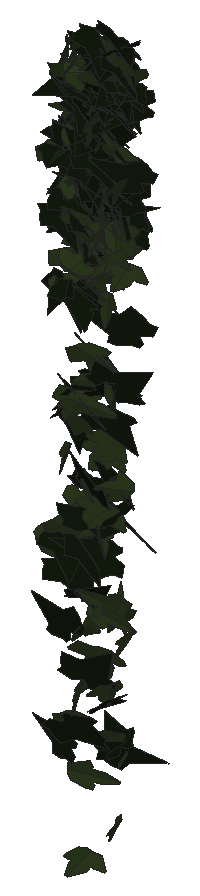
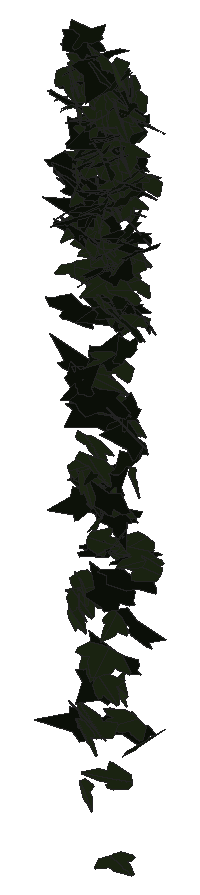
# SketchUp Ruby script. Lengths in millimetres.
U = 1.mm
M = Sketchup.active_model
def pt(a) = Geom::Point3d.new(a.map { |v| v * U })
def face(e, loops, mat)
  f = e.add_face(loops[0].map { |a| pt(a) })
  loops[1..].each { |l| e.add_face(l.map { |a| pt(a) }).erase! }
  f.material = f.back_material = mat if mat
  f
end
# faces: each face lists its corners as indices into pts; further lists are holes
def faces(e, pts, list, mat = nil) = list.each { |f| face(e, (f[0].is_a?(Array) ? f : [f]).map { |l| l.map { |i| pts[i] } }, mat) }
# xy, xz, yz: faces in a plane at the given z, y or x. An outline is a flat list of corners, or four numbers for a rectangle; further outlines are holes
def ring(l) = l.size == 4 ? [[l[0], l[1]], [l[2], l[1]], [l[2], l[3]], [l[0], l[3]]] : l.each_slice(2).to_a
def flat(e, list, mat, &to3) = list.each { |f| face(e, (f[0].is_a?(Array) ? f : [f]).map { |l| ring(l).map { |u, v| to3.(u, v) } }, mat) }
def xy(e, z, list, mat = nil) = flat(e, list, mat) { |x, y| [x, y, z] }
def xz(e, y, list, mat = nil) = flat(e, list, mat) { |x, z| [x, y, z] }
def yz(e, x, list, mat = nil) = flat(e, list, mat) { |y, z| [x, y, z] }
def lines(e, pts, list) = list.each { |a, b| e.add_line(pt(pts[a]), pt(pts[b])) }
# prism: a flat outline (further loops are holes) pulled along v
def prism(e, loops, v, mat = nil)
  f = face(e, loops, mat); d = Geom::Vector3d.new(v.map { |x| x * U })
  f.pushpull(f.normal.samedirection?(d) ? d.length : -d.length)
end
def box(e, o, s, mat = nil) = prism(e, [[o, [o[0] + s[0], o[1], o[2]], [o[0] + s[0], o[1] + s[1], o[2]], [o[0], o[1] + s[1], o[2]]]], [0, 0, s[2]], mat)
def at(x, y, z, deg = 0) = Geom::Transformation.translation(pt([x, y, z])) * Geom::Transformation.rotation(ORIGIN, Z_AXIS, deg.degrees)
def axes(o, x, y, z) = Geom::Transformation.new([*x, 0, *y, 0, *z, 0, *pt(o).to_a, 1])
def part(name) = M.definitions.add(name)
# library, detail: a bought-in or finely detailed component or shape, given as its bounding box
def library(name, o, s) = part(name).tap { |d| box(d.entities, o, s) }
def detail(e, o, s) = box(e.add_group.entities, o, s)
def put(e, d, t, mat = nil) = e.add_instance(d, t).tap { |i| i.material = mat if mat }
def group(e, t, mat = nil) = e.add_group.tap { |g| g.transformation = t; g.material = mat if mat }.entities
root = M.entities
M.materials.add("efeu1").color = [18, 25, 13]
M.materials.add("efeu2").color = [43, 57, 29]
c1 = part("ivyleaf_10")
p = [[0,12.8,-0.8],[-1.5,51.3,-10.9],[-4.9,51,-11.6],[-13.6,26.5,-7.3],[-13.2,15.9,-4.6],[-21.1,19.3,-7.2],
  [-29.5,16.3,-8.3],[-29.2,8.3,-6.2],[-19.7,-9.8,0.5],[-7.6,-13,4],[1,-12.2,5.8],[-0.4,51.1,-11.1],
  [-1.5,51.1,-10.9],[1,-12.4,5.9],[16.9,-12.4,3.5],[35.1,9.1,-5.1],[35,12.9,-6.1],[20.5,16.4,-4.9],
  [15.8,15,-3.8],[15.3,27.6,-7.1],[12.8,31.3,-7.8]]
faces(c1.entities,p,[[0,1,2,3,4,5,6,7,8,9,10],[11,12,0,13,14,15,16,17,18,19,20]],"efeu2")
c2 = part("ivyleaf_9")
p = [[39.1,54.8,31.7],[34.5,51.8,30.2],[-5.3,25.2,17.3],[-17.9,28.3,20.9],[-21.6,21.7,17],[-20.2,4.3,5.3],
  [-22.9,-0.3,2.5],[-17.1,-4,-0.6],[-2,-2.1,-1.2],[-0.7,-15.4,-10.1],[16.6,-22.3,-16.7],[21.1,-15.1,-12.5],
  [32.7,-10.7,-11],[46.1,-1.8,-6.6],[30.8,11.2,3.8]]
faces(c2.entities,p,[[0,1,2,3,4,5,6,7,8,9,10,11,12,13,14]],"efeu1")
put(root,c1,axes([2423.7,959.7,428.7],[0.42918,-0.51053,0.64216],[0.55619,-0.57229,-0.55762],[1.4589,0.36837,0.02368]))
put(root,c1,axes([2519.9,950.3,1384],[0.10116,-0.81817,0.0626],[-0.0042,-0.06288,-0.81987],[1.56168,0.05283,-0.00626]))
put(root,c1,axes([2466.4,955.7,1470.6],[0.11764,-0.75177,0.34655],[0.10851,-0.34282,-0.75385],[1.57173,0.07993,0.02611]))
put(root,c1,axes([2417.6,948.7,1568.5],[0.34944,-0.81684,-0.06645],[-0.02225,0.06548,-0.83722],[1.55959,0.18395,0.00295]))
put(root,c1,axes([2484,949.2,779.4],[1.57579,-0.10908,-0.34609],[-0.65321,0.04451,-0.83512],[0.22422,0.89629,-0.00065]))
put(root,c2,axes([2498.1,963.2,1633.7],[-0.17423,-0.67542,0.52153],[0.47468,-0.5228,-0.63328],[1.55316,0.08401,0.25205]))
put(root,c2,axes([2432.3,955.2,696.6],[0.16667,-0.81995,-0.11019],[-0.02639,0.10933,-0.82461],[1.57434,0.08864,-0.00216]))
put(root,c2,axes([2431,945.6,1418.8],[-0.93455,0.09387,0.70212],[1.23515,-0.28279,0.49169],[0.54033,0.80878,0.09043]))
put(root,c2,axes([2453.5,951.6,1417.3],[0.09734,-0.79256,-0.34222],[0.10732,0.34515,-0.79093],[1.63949,0.02446,0.07209]))
put(root,c2,axes([2457.5,943.1,740.9],[-1.30236,0.01154,0.54128],[1.03011,-0.00582,0.68439],[0.0241,0.87248,-0.00259]))
put(root,c1,axes([2378.7,944.8,1402.3],[-0.69228,-0.44049,-0.55113],[1.01872,0.23167,-0.53843],[0.87478,-0.61838,0.19087]))
put(root,c2,axes([2395.2,960.7,689.2],[-0.40626,-0.83532,-0.06765],[0.01712,0.06753,-0.86213],[1.5949,-0.2135,-0.00798]))
put(root,c2,axes([2391.9,946,1405.4],[0.10948,-0.47721,-0.63361],[0.10888,0.63611,-0.4739],[1.50571,-0.0113,0.08034]))
put(root,c2,axes([2463,949.2,798.5],[0.52534,-0.53448,0.66931],[-0.43549,0.63163,0.59876],[-1.5709,-0.35384,0.05784]))
put(root,c2,axes([2443.5,948.4,460.5],[-0.91593,0.14357,0.66024],[1.12315,-0.30542,0.49658],[0.62621,0.75779,0.07505]))
put(root,c1,axes([2472.4,954.6,734.5],[-0.10834,0.7349,-0.30371],[0.05244,-0.30248,-0.73709],[-1.51248,-0.06313,-0.0038]))
put(root,c2,axes([2391.5,957.8,1156.9],[-1.14108,0.14142,-0.49329],[0.89744,-0.14744,-0.6154],[-0.38528,-0.76228,0.02751]))
put(root,c1,axes([2404.9,961.3,1356.8],[0.27602,-0.50452,0.59318],[1.0173,-0.37428,-0.44903],[1.07776,0.4825,0.27193]))
put(root,c2,axes([2425.7,958.2,1153],[-0.68074,-0.70087,-0.2783],[0.22525,0.25203,-0.78682],[1.41742,-0.37666,-0.00862]))
put(root,c1,axes([2425.3,947,927.3],[-1.31838,0.29849,0.21379],[-0.37768,0.07971,-0.75428],[-0.58792,-0.72056,0.00512]))
put(root,c2,axes([2463,963.2,1620.2],[-0.43825,-0.82502,0.03105],[-0.0162,-0.02986,-0.85655],[1.5712,-0.23043,-0.00017]))
put(root,c1,axes([2477.4,960,1153.1],[1.04945,-0.44206,0.40539],[0.56454,-0.27763,-0.70622],[0.99216,0.62555,-0.02696]))
put(root,c2,axes([2403.1,957.8,317.2],[-0.23314,-0.79978,0.1421],[0.04083,0.14047,0.80911],[-1.54544,0.12436,-0.00006]))
put(root,c2,axes([2415.9,942.2,540.3],[-0.18859,0.13593,0.84531],[-0.87282,0.71015,-0.16795],[-1.37598,-0.4691,-0.00932]))
put(root,c1,axes([2520.4,950.6,1287.2],[1.16434,-0.44278,-0.34263],[-0.48377,0.23253,-0.75435],[0.94939,0.66152,0.03583]))
put(root,c1,axes([2509.7,965.4,816.4],[0.0865,0.23688,0.7628],[-0.26221,-0.75026,0.24119],[1.49736,-0.14506,-0.00183]))
put(root,c1,axes([2465,960.9,1303.9],[-0.40203,0.57267,-0.58428],[0.24087,-0.57331,-0.60767],[-1.53832,-0.23943,0.05755]))
put(root,c1,axes([2489.5,951,457.1],[-0.56264,-0.72009,-0.13796],[0.1065,0.12615,-0.7784],[1.39133,-0.30085,0.00379]))
put(root,c1,axes([2461.3,952,1485.8],[0.26626,-0.80695,-0.17252],[-0.0737,0.16837,-0.81893],[1.56876,0.14487,-0.00919]))
put(root,c1,axes([2445.5,960.7,1392.9],[0.75294,-0.71526,0.2599],[0.22999,-0.23016,-0.81736],[1.42998,0.41363,-0.00538]))
put(root,c1,axes([2399,955.6,1208.1],[-1.06414,-0.23857,-0.44204],[0.94713,-0.17329,-0.53596],[0.1298,-0.69137,0.28686]))
put(root,c2,axes([2517,941.3,782.8],[-0.34441,0.76154,0.32734],[-0.15165,0.31752,-0.78274],[-1.57028,-0.19769,0.0038]))
put(root,c1,axes([2457.3,961.4,1269.3],[0.82671,-0.61985,0.27564],[0.28301,-0.23234,-0.75682],[1.25968,0.459,-0.01087]))
put(root,c1,axes([2438.7,958.6,1473.2],[0.78386,-0.70817,0.08456],[0.0753,-0.07481,-0.81922],[1.35528,0.41374,-0.00339]))
put(root,c1,axes([2399.7,946,1405.5],[-0.13178,-0.61189,-0.50447],[0.12519,0.50021,-0.61575],[1.50409,-0.09524,0.00705]))
put(root,c1,axes([2485.9,958,1248.8],[0.84377,-0.22823,-0.69233],[1.21346,-0.27142,0.49776],[-0.67257,-0.77602,0.02952]))
put(root,c2,axes([2495.2,953,1000.4],[-0.60385,0.19408,0.80129],[1.31944,-0.40187,0.37185],[0.84922,0.76239,-0.00797]))
put(root,c2,axes([2500.2,966.4,1390.4],[-0.66734,0.06385,0.72928],[-1.15355,-0.47881,-0.2495],[0.78138,-0.65234,0.25451]))
put(root,c1,axes([2429,947.1,958.8],[-0.67269,-0.24827,-0.7794],[1.36217,0.3172,-0.42562],[0.75372,-0.79484,0.0736]))
put(root,c2,axes([2406.8,955.6,646.1],[-0.62425,-0.47585,-0.61472],[0.64503,0.51292,-0.57789],[1.3315,-0.47157,-0.00825]))
put(root,c1,axes([2419.8,963.3,1354.4],[0.11933,-0.74217,0.31287],[0.00074,-0.31379,-0.74442],[1.53287,0.05793,-0.024]))
put(root,c1,axes([2424.6,946.8,1202.8],[0.99733,0.27008,-0.47127],[0.68938,0.31422,0.58285],[0.77036,-0.63085,0.08854]))
put(root,c2,axes([2514.5,949,1626.2],[-0.04872,0.82399,-0.17062],[-0.02885,-0.17112,-0.82414],[-1.60122,-0.02199,0.02004]))
put(root,c2,axes([2403.7,969.9,952.3],[0.53392,-0.58906,0.69287],[0.5142,-0.63837,-0.65211],[1.65268,0.38892,-0.02095]))
put(root,c1,axes([2474.2,957.7,1611.6],[1.37264,-0.45576,-0.02408],[0.03134,0.07099,-0.85039],[0.86805,0.71813,0.06878]))
put(root,c1,axes([2501.8,958.1,212.5],[0.25989,-0.72766,-0.02306],[-0.00904,0.02257,-0.74036],[1.38554,0.13664,-0.0005]))
put(root,c2,axes([2452.4,966.5,1040.7],[0.95655,-0.66038,0.08772],[-0.09983,0.07031,0.82988],[-1.26393,-0.50533,0.00084]))
put(root,c2,axes([2405.7,948.5,365.1],[0.03186,-0.05946,-0.84196],[0.79779,0.73152,-0.04333],[1.39431,-0.4172,0.04403]))
put(root,c2,axes([2440.7,965.6,1376.1],[-0.18211,-0.80257,-0.06848],[0.01284,0.06816,-0.80825],[1.53294,-0.09592,-0.00137]))
put(root,c1,axes([2495.1,964.7,598.8],[-0.66578,-0.1313,-0.77141],[-1.36751,-0.28073,0.37362],[-0.58978,0.79915,0.00451]))
put(root,c2,axes([2376.4,961.5,1277.4],[0.16897,-0.78102,-0.2264],[0.00336,0.22793,-0.7856],[1.54762,0.08478,0.02643]))
put(root,c1,axes([2412.3,949.7,1559.7],[-1.04274,-0.30516,-0.59299],[0.94873,0.32242,-0.6265],[0.84315,-0.74018,-0.02842]))
put(root,c1,axes([2465.8,955.9,586],[0.43635,0.05961,0.75663],[1.39767,0.18218,-0.23688],[-0.36478,0.76933,-0.00253]))
put(root,c1,axes([2396.9,963.7,952.3],[1.11663,-0.49198,0.27184],[0.4082,-0.16726,-0.76563],[0.98882,0.62462,0.00909]))
put(root,c1,axes([2472.6,959.1,1448.9],[0.37516,-0.7967,-0.07406],[0.00366,0.07674,-0.82048],[1.52282,0.19609,0.02022]))
put(root,c2,axes([2439.2,975.7,1340.3],[-0.69506,-0.47282,0.58309],[0.08582,-0.66108,-0.50781],[1.42616,-0.19065,0.31474]))
put(root,c1,axes([2422.6,945.4,1553.1],[0.24007,-0.20221,-0.804],[1.05841,0.62378,-0.06963],[1.17017,-0.52272,0.22793]))
put(root,c1,axes([2500.6,943,986.8],[0.05595,0.29057,-0.75135],[0.04598,0.75119,0.29146],[1.53248,-0.03315,0.01869]))
put(root,c2,axes([2422.6,968.9,1525.5],[-1.56669,-0.03754,0.13475],[-0.22639,-0.23536,-0.79225],[0.14008,-0.80025,0.22668]))
put(root,c1,axes([2406.4,956,371.8],[-1.08412,-0.02773,-0.54153],[1.02893,0.03134,-0.57029],[0.07934,-0.78533,-0.00364]))
put(root,c2,axes([2427.4,966,1321.8],[1.10109,-0.08826,-0.5894],[1.12859,0.00323,0.58159],[-0.11325,-0.8259,0.06526]))
put(root,c1,axes([2418.1,950.4,1348.9],[0.53932,0.58866,0.45523],[0.38345,0.40824,-0.65331],[-1.36337,0.34768,-0.00366]))
put(root,c1,axes([2478.9,967.2,1004.2],[-0.51878,-0.19184,0.73741],[-1.06838,-0.47901,-0.33213],[0.98058,-0.6234,0.02827]))
put(root,c2,axes([2477.2,973.3,680.7],[-0.51033,-0.72491,-0.50906],[-0.30861,-0.48271,0.77281],[-1.65736,0.3131,0.01285]))
put(root,c2,axes([2538.3,967.9,1384.2],[-0.22028,0.10753,0.7993],[-1.47639,-0.23573,-0.08062],[0.41988,-0.77247,0.13587]))
put(root,c2,axes([2407.7,957,1519.8],[1.14384,0.32484,-0.52857],[0.84484,0.28896,0.68233],[0.82489,-0.74639,0.03411]))
put(root,c1,axes([2424.9,965.6,1607.1],[0.29135,-0.82908,0.14199],[0.02122,-0.14231,-0.84297],[1.60074,0.15278,-0.01467]))
put(root,c2,axes([2535.2,963.7,1108.4],[-0.4443,0.03377,0.87946],[-1.63582,0.18695,-0.23533],[-0.36026,-0.8905,-0.01605]))
put(root,c1,axes([2399.1,956.6,1585.3],[0.35,-0.76296,-0.31972],[0.12851,0.34027,-0.77318],[1.56915,0.14231,0.13464]))
put(root,c1,axes([2363.4,956.9,672.7],[0.42259,0.02958,-0.80727],[1.53113,0.06762,0.22376],[0.13904,-0.83452,-0.01049]))
put(root,c2,axes([2487.3,954.6,1347],[-0.46175,-0.03034,0.81647],[1.55435,0.01516,0.24325],[-0.04412,0.85162,0.02476]))
put(root,c1,axes([2466.9,960.8,1551.8],[-1.17324,-0.53676,-0.00082],[0.00215,-0.00005,-0.81739],[1.02155,-0.61646,0.00078]))
put(root,c1,axes([2385.2,952.8,719.7],[-0.61484,-0.34149,-0.58795],[0.78453,0.4193,-0.47003],[1.0291,-0.52368,0.00705]))
put(root,c2,axes([2427.4,962.7,595.2],[1.28917,0.39988,0.1042],[-0.17142,-0.0524,0.7866],[0.76756,-0.68333,0.00066]))
put(root,c2,axes([2448.1,976.2,1444.8],[-0.89218,-0.60321,0.25493],[-0.17026,-0.25158,-0.7598],[1.23465,-0.47058,0.07943]))
put(root,c1,axes([2496.6,965.1,1587.4],[-0.98113,0.48018,-0.43412],[0.5512,-0.32524,-0.70366],[-1.10181,-0.59029,0.03456]))
put(root,c1,axes([2425.1,968.8,1270.1],[-0.56587,-0.25344,0.69395],[-1.0652,-0.411,-0.3899],[0.91778,-0.63328,-0.02467]))
put(root,c1,axes([2447.8,967.9,1218.5],[0.78957,-0.34005,-0.64694],[1.02551,-0.36029,0.53491],[-0.93977,-0.67885,0.04017]))
put(root,c2,axes([2426,960.4,1494.9],[1.04894,-0.55181,-0.28459],[-0.26114,0.26288,-0.77544],[1.15243,0.56182,0.08331]))
put(root,c2,axes([2493.7,969.8,1592.9],[0.18396,-0.82403,-0.08937],[-0.00172,0.08987,-0.82962],[1.57748,0.09619,0.00952]))
put(root,c2,axes([2443.5,956.8,757.4],[0.69928,0.04049,-0.70012],[-1.3299,-0.04581,-0.36936],[-0.11305,0.78935,0.01447]))
put(root,c1,axes([2392,964,1257.9],[-0.35439,0.06267,-0.81817],[1.51136,-0.19756,-0.19586],[-0.39337,-0.81551,-0.01542]))
put(root,c1,axes([2432,959.1,1044.5],[-1.04584,-0.12956,-0.59148],[1.114,0.09081,-0.56369],[0.295,-0.80223,0.03172]))
put(root,c1,axes([2513.6,958,1287.7],[1.15367,-0.46995,0.37037],[-0.56769,0.21971,0.76696],[-0.9872,-0.67554,-0.00821]))
put(root,c1,axes([2472.8,956.4,1368.2],[0.27613,-0.66521,-0.44848],[-0.00645,0.45525,-0.67634],[1.52687,0.12223,0.07825]))
put(root,c1,axes([2491.5,954.8,1275.9],[0.51745,-0.2591,-0.81608],[-1.11332,0.56904,-0.37556],[1.18996,0.64506,0.0035]))
put(root,c1,axes([2469.8,958.8,1448],[-1.03535,0.12691,0.70025],[-1.32842,0.07673,-0.55616],[-0.26412,-0.8834,0.05229]))
put(root,c2,axes([2509.2,974.2,1552.1],[-1.35212,-0.41412,0.06534],[-0.08846,-0.04997,-0.82209],[0.79299,-0.71169,0.0197]))
put(root,c1,axes([2465.8,976.1,1270.6],[-0.22825,-0.561,0.57544],[0.10775,-0.58626,-0.55975],[1.5257,-0.04252,0.12562]))
put(root,c2,axes([2478.3,978.5,1495.8],[-1.0494,-0.59264,0.17754],[0.04749,-0.25893,-0.78683],[1.17648,-0.51817,0.19012]))
put(root,c2,axes([2438.4,976.2,1476.6],[-0.86031,-0.66334,0.09907],[-0.10556,-0.08209,-0.80272],[1.2721,-0.45542,0.00039]))
put(root,c1,axes([2439.8,953.3,551.7],[-0.35687,-0.53461,-0.62944],[0.36319,0.59995,-0.56641],[1.52919,-0.26725,-0.01237]))
put(root,c2,axes([2421.6,962.4,1145.7],[1.47936,-0.31884,0.07692],[0.13626,-0.02813,-0.84015],[0.60917,0.78059,0.00114]))
put(root,c1,axes([2487.4,978.6,1210.4],[-0.11234,-0.28963,0.71903],[-0.21253,-0.71041,-0.29532],[1.45991,-0.1257,0.01234]))
put(root,c1,axes([2387.7,972.1,844.4],[0.59581,-0.65939,0.28538],[0.2884,-0.2437,-0.72931],[1.33669,0.34649,0.03015]))
put(root,c2,axes([2483.7,978,1534.7],[0.11047,-0.7547,0.31294],[0.18156,-0.30532,-0.75402],[1.54429,0.08988,0.06626]))
put(root,c1,axes([2422.5,965.2,1238.5],[-0.28326,0.72588,-0.13156],[0.04795,-0.12913,-0.74098],[-1.40319,-0.15095,0.00124]))
put(root,c1,axes([2491.5,972.7,1352.1],[0.44707,0.59012,-0.50006],[-0.5733,-0.41156,-0.62718],[-1.3559,0.36859,0.1003]))
put(root,c1,axes([2365.7,958.3,695.5],[0.77314,0.38699,0.6006],[0.84235,0.40606,-0.56101],[-1.06748,0.60071,-0.0077]))
put(root,c1,axes([2511.9,973.5,546.2],[0.18937,-0.7101,0.29811],[0.05543,-0.2969,-0.71694],[1.46467,0.10304,-0.01141]))
put(root,c1,axes([2482.9,971.6,1262.9],[0.41465,-0.73463,0.17048],[0.04992,-0.16996,-0.76593],[1.43444,0.21827,-0.02263]))
put(root,c2,axes([2486.3,958.3,1327.3],[0.94681,-0.25214,-0.63948],[-1.08534,0.28935,-0.55773],[0.73044,0.75677,0.00019]))
put(root,c2,axes([2490.2,962.6,1576.9],[-0.84743,0.69545,-0.09822],[0.0849,-0.08806,-0.82572],[-1.33401,-0.44739,0.00984]))
put(root,c2,axes([2465.1,960.7,1590.1],[-0.80186,0.70206,0.02308],[-0.01398,0.02251,-0.81876],[-1.33681,-0.42135,-0.00528]))
put(root,c1,axes([2448.8,953,790.6],[-0.08488,0.3922,-0.6869],[-0.34761,0.66429,0.39115],[1.46472,0.18038,0.05302]))
put(root,c1,axes([2432.9,971.7,1460.5],[1.03647,-0.59183,0.15873],[0.22758,-0.10563,-0.8041],[1.14376,0.55733,0.01615]))
put(root,c2,axes([2372.9,968.3,1514.4],[1.07995,-0.60299,-0.06393],[-0.0763,0.05006,-0.82798],[1.15152,0.56883,0.0051]))
put(root,c1,axes([2405.6,973.2,744.2],[-0.15075,0.63149,-0.46442],[0.13523,-0.45908,-0.63634],[-1.48573,-0.10586,-0.0108]))
put(root,c1,axes([2413.3,953.7,1437.5],[0.20301,0.64739,0.59586],[0.12099,0.59298,-0.65564],[-1.67018,0.12165,0.02493]))
put(root,c1,axes([2417.6,963,763.4],[1.09639,-0.06691,-0.43727],[0.84178,0.09879,0.56759],[0.01368,-0.71646,0.1191]))
put(root,c2,axes([2416.2,978.1,1588.8],[0.34433,-0.79373,0.16353],[0.01497,-0.16583,-0.81359],[1.54229,0.17882,-0.02861]))
put(root,c1,axes([2428.5,969.3,1238.4],[1.14301,0.41047,-0.19109],[-0.36523,-0.05674,-0.72501],[-0.78049,0.62768,0.05942]))
put(root,c2,axes([2411.6,979.8,1223.8],[-0.04461,-0.27847,0.74599],[0.6707,-0.67287,-0.2401],[1.35897,0.32294,0.14299]))
put(root,c1,axes([2497.8,954.2,1282.7],[0.23198,0.57494,0.68034],[0.26356,0.6661,-0.58771],[-1.67464,0.18448,0.00175]))
put(root,c2,axes([2435.7,977.9,1523.6],[0.0898,-0.829,0.02894],[-0.03835,-0.03012,-0.83005],[1.57824,0.04644,-0.02181]))
put(root,c1,axes([2443.4,968.8,1489.3],[1.43524,-0.21779,-0.249],[-0.42861,0.11603,-0.78355],[0.46117,0.78564,0.04669]))
put(root,c2,axes([2538.1,964,1354.4],[-1.17079,0.45173,0.46743],[-0.71648,0.27706,-0.76321],[-1.00856,-0.72122,-0.00043]))
put(root,c2,axes([2467.8,953.3,988.1],[0.9875,0.45925,0.48026],[0.69854,0.30987,-0.69285],[-1.05425,0.63549,-0.00923]))
put(root,c1,axes([2398.6,971.7,1199],[0.90906,-0.02765,0.635],[1.20491,-0.0497,-0.47838],[0.10721,0.79303,-0.00784]))
put(root,c2,axes([2429.9,983,1481.2],[-0.63605,-0.69655,0.2395],[-0.07053,-0.24677,-0.76939],[1.40008,-0.32887,0.07005]))
put(root,c2,axes([2441.6,984.1,1327.6],[0.19879,-0.27062,-0.74441],[1.09712,-0.48897,0.25864],[-1.03383,-0.57094,0.13134]))
put(root,c1,axes([2462.8,971.3,340.1],[-1.3241,-0.09009,0.43905],[0.83887,0.0095,0.70039],[-0.15469,0.82262,0.04]))
put(root,c2,axes([2408.5,969.6,1385.5],[0.16837,-0.69389,-0.44416],[-0.01617,0.44592,-0.69833],[1.56791,0.07911,0.0405]))
put(root,c2,axes([2466.3,969.2,938],[-0.53097,-0.26925,-0.74167],[1.05463,0.49316,-0.38748],[1.06904,-0.62025,0.01388]))
put(root,c2,axes([2472.4,953.5,417.2],[0.58584,0.53031,0.49446],[0.43879,0.4377,-0.61297],[-1.30832,0.38426,0.01583]))
put(root,c2,axes([2406.6,966.1,1555.5],[1.4752,-0.32673,-0.013],[0.06231,0.11084,-0.83328],[0.61919,0.76726,0.11484]))
put(root,c1,axes([2501.1,976.8,584.6],[-0.41648,-0.68094,0.3041],[-0.16772,-0.2911,-0.71522],[1.40938,-0.23586,0.00475]))
put(root,c2,axes([2468.3,961.3,1311.9],[0.47649,-0.00027,0.79652],[1.48185,0.17616,-0.24467],[-0.31969,0.81615,0.05308]))
put(root,c1,axes([2460.2,971.1,1491.3],[-0.24893,-0.81296,-0.08467],[0.18339,0.06981,-0.81916],[1.54475,-0.1393,0.08361]))
put(root,c2,axes([2430.1,979.7,1282.2],[-1.43242,-0.21323,0.16253],[-0.29303,-0.05276,-0.78221],[0.41774,-0.76818,0.00861]))
put(root,c2,axes([2490.1,973.1,762.4],[1.14796,-0.5162,0.04875],[0.0702,-0.03188,-0.7939],[0.98431,0.6043,-0.00024]))
put(root,c1,axes([2464.8,971.7,1571.3],[-0.67073,-0.76911,-0.03582],[0.02382,0.03367,-0.846],[1.46516,-0.35264,-0.00264]))
put(root,c1,axes([2471.7,972.2,1419.4],[1.52225,0.16606,0.22125],[0.41085,0.04862,-0.81689],[-0.32924,0.82845,0.00359]))
put(root,c1,axes([2460,968.6,1487.8],[-1.53667,-0.01746,-0.16808],[0.31908,0.01997,-0.80745],[0.04028,-0.82448,-0.016]))
put(root,c2,axes([2489.9,960.3,339.1],[0.48114,0.19222,-0.71859],[0.4837,0.69096,0.27424],[1.3305,-0.32071,0.16016]))
put(root,c2,axes([2493,978.6,1531],[0.31268,-0.81077,-0.06081],[-0.04539,0.05721,-0.82716],[1.54672,0.16558,-0.01198]))
put(root,c2,axes([2511.3,986.3,1315.1],[-0.25206,-0.68712,0.35712],[-0.14259,-0.34923,-0.69973],[1.46689,-0.15202,-0.00666]))
put(root,c1,axes([2476.4,973.2,887.2],[1.42237,-0.32915,-0.18532],[-0.32243,0.07511,-0.81663],[0.64255,0.76632,0.00045]))
put(root,c2,axes([2454.7,975.9,1510.9],[0.89205,-0.68381,0.0131],[0.07018,0.00941,-0.82826],[1.29978,0.4688,0.03573]))
put(root,c2,axes([2420.4,980.7,1159],[0.55601,-0.6095,0.36994],[0.47193,-0.28798,-0.67028],[1.27225,0.37319,0.08696]))
put(root,c2,axes([2444,982.3,1349.8],[0.34916,-0.44461,0.62928],[0.71188,-0.51415,-0.47231],[1.28204,0.40658,0.09088]))
put(root,c2,axes([2462.5,976.2,834.5],[0.77343,-0.67778,-0.04257],[-0.04552,0.0353,-0.79027],[1.2917,0.40708,-0.00236]))
put(root,c1,axes([2488.3,958.8,1466.7],[0.12507,0.58553,0.60075],[-0.1997,0.6036,-0.57682],[-1.58404,-0.02987,0.12015]))
put(root,c1,axes([2505.7,977.1,1209.7],[0.90542,0.52141,-0.33208],[-0.47053,-0.22359,-0.70524],[-1.07833,0.53536,0.02889]))
put(root,c2,axes([2478.7,975.4,1344.9],[-0.89056,0.18813,0.62786],[-1.20612,0.06703,-0.49239],[-0.31837,-0.78018,0.1091]))
put(root,c2,axes([2494.7,964.8,1449.1],[-0.37295,-0.34475,0.75162],[1.11833,0.48542,0.37585],[-1.10729,0.60638,0.12644]))
put(root,c2,axes([2395,974.8,1306.8],[-0.31578,-0.62665,-0.45932],[0.19767,0.44757,-0.64814],[1.46544,-0.19541,-0.01155]))
put(root,c1,axes([2429.5,977.4,1523.8],[-0.88949,-0.64643,0.18683],[-0.14361,-0.17569,-0.79664],[1.27256,-0.47166,0.04069]))
put(root,c1,axes([2382.4,969.7,1149],[0.7676,0.56558,0.24405],[0.30243,0.18631,-0.69437],[-1.13267,0.43303,-0.02001]))
put(root,c1,axes([2453,986.7,712],[-0.15849,-0.26911,0.71982],[-0.47191,-0.67591,-0.28138],[1.38436,-0.26122,-0.01351]))
put(root,c1,axes([2391.3,972.2,1513.3],[0.98729,-0.04959,0.64712],[1.20901,0.20854,-0.49325],[-0.25309,0.80273,0.16812]))
put(root,c1,axes([2413.2,973.1,1371.4],[-1.29842,-0.41201,-0.00439],[0.00522,0.00396,-0.79699],[0.78417,-0.68223,-0.00197]))
put(root,c2,axes([2382.4,984.9,1412.1],[0.26184,-0.75271,0.21451],[0.19339,-0.19877,-0.76268],[1.47699,0.15947,0.06184]))
put(root,c2,axes([2448.6,977.8,1226.7],[0.17281,-0.72471,-0.26389],[-0.04132,0.2632,-0.7303],[1.46727,0.09277,0.01051]))
put(root,c2,axes([2418.7,978.6,1275.3],[0.33014,-0.76248,-0.20975],[-0.01828,0.21269,-0.78111],[1.50495,0.16985,0.03653]))
put(root,c1,axes([2421.9,980.6,114.8],[0.8627,0.48758,-0.45262],[-0.6355,-0.30698,-0.66509],[-1.09514,0.56223,0.02939]))
put(root,c1,axes([2518.8,975.8,1568.5],[-0.69371,-0.74114,0.00565],[-0.00599,-0.00475,-0.82592],[1.41056,-0.36451,-0.00073]))
put(root,c1,axes([2414.2,976.4,1539.3],[0.41931,-0.80028,-0.06678],[-0.02638,0.06545,-0.83005],[1.52817,0.22072,0.00399]))
put(root,c1,axes([2455.6,965.1,1189.1],[-0.50701,-0.34579,-0.60588],[0.66795,0.49407,-0.43629],[1.14743,-0.4404,-0.01374]))
put(root,c1,axes([2444.1,978.6,1279.5],[-1.40673,0.10485,0.29304],[0.53779,-0.09043,0.74509],[0.24827,0.78995,0.0464]))
put(root,c1,axes([2460.5,958.5,1249.1],[0.0451,-0.15167,0.87928],[-0.05083,0.87908,0.15235],[-1.6974,-0.03036,0.0188]))
put(root,c1,axes([2408.8,977.2,1468.2],[-1.21901,-0.45772,0.15302],[-0.17283,-0.13544,-0.78522],[0.90211,-0.64445,0.05634]))
put(root,c1,axes([2469.6,978.1,1554.3],[-1.30688,-0.27736,0.36474],[-0.57626,-0.21857,-0.73623],[0.65458,-0.74618,0.08008]))
put(root,c2,axes([2476.7,982,1382.4],[-1.3462,-0.01372,-0.3327],[0.6337,-0.03678,-0.70638],[-0.0062,-0.7808,0.03912]))
put(root,c1,axes([2491.2,970,590.1],[0.88696,-0.61961,0.37531],[-0.4296,0.29984,0.77531],[-1.31006,-0.51782,-0.00015]))
put(root,c1,axes([2508.2,975.1,1533.2],[0.36956,-0.7978,-0.16362],[-0.00911,0.16709,-0.82038],[1.54995,0.1912,0.03419]))
put(root,c2,axes([2503.7,962.4,351.7],[-1.17755,0.31415,-0.51079],[-0.86839,0.22961,0.69391],[0.74057,0.76877,0.00148]))
put(root,c1,axes([2493,988.8,1379.5],[-0.10449,0.31499,-0.746],[0.07336,-0.74585,-0.31776],[-1.53942,-0.05692,0.03549]))
put(root,c2,axes([2401.8,986,1408],[0.25323,-0.79394,0.12439],[-0.00327,-0.12636,-0.8047],[1.52945,0.13118,-0.02231]))
put(root,c2,axes([2453.8,980.9,1446.9],[0.58638,-0.73797,-0.06503],[-0.01315,0.06756,-0.79947],[1.40989,0.30756,0.01959]))
put(root,c2,axes([2448.6,971.2,1472.3],[1.29136,-0.34345,-0.31279],[-0.45021,0.22106,-0.75588],[0.76088,0.71369,0.08361]))
put(root,c2,axes([2388.6,992,1315.7],[-0.46933,-0.13898,0.76089],[-0.35589,-0.76422,-0.2002],[1.42842,-0.23607,0.20012]))
put(root,c2,axes([2514.2,982.8,1282.2],[-1.37278,-0.06709,-0.23637],[0.45095,0.0041,-0.72421],[0.12378,-0.75903,0.01699]))
put(root,c2,axes([2436.2,991.3,1384.4],[-1.00038,-0.56705,0.21694],[-0.04104,-0.26933,-0.75623],[1.15476,-0.50081,0.16106]))
put(root,c1,axes([2438.9,988.3,1270.6],[0.40692,-0.30403,0.73736],[1.101,-0.46643,-0.36006],[1.04499,0.60981,0.09223]))
put(root,c2,axes([2482.4,979.4,1554.3],[0.44572,-0.74444,-0.2667],[0.10391,0.29271,-0.7691],[1.50141,0.20074,0.1324]))
put(root,c2,axes([2538.5,978.2,1519.4],[-1.284,0.34949,0.34378],[-0.70002,0.02578,-0.74802],[-0.61683,-0.75676,0.13328]))
put(root,c1,axes([2397.9,982.3,1459.5],[0.5447,-0.75883,0.13365],[0.13858,-0.11529,-0.81055],[1.45987,0.29407,0.02708]))
put(root,c2,axes([2422.8,988.1,1444.2],[-0.34916,-0.78927,0.02669],[-0.01423,-0.02566,-0.81031],[1.50292,-0.18361,-0.00147]))
put(root,c2,axes([2427.7,978.9,961.2],[-1.34498,0.43793,-0.15557],[0.25278,-0.08101,-0.83138],[-0.8476,-0.71906,-0.00108]))
put(root,c2,axes([2426.3,980.3,781],[-0.28342,0.12526,0.76329],[1.04641,-0.5296,0.19418],[1.03546,0.56949,0.01269]))
put(root,c2,axes([2388.5,988.6,1419.3],[0.3268,-0.75603,0.22366],[0.0838,-0.21935,-0.77527],[1.49818,0.17718,-0.00542]))
put(root,c1,axes([2405.2,979.5,1533.1],[-0.62435,-0.75834,0.01412],[-0.00791,-0.01359,-0.82625],[1.44349,-0.32808,0.00158]))
put(root,c2,axes([2396.6,988.2,1410.1],[-1.31815,-0.32698,-0.26214],[0.58441,-0.05135,-0.74726],[0.5428,-0.73876,0.16797]))
put(root,c2,axes([2443.8,975.8,1367.2],[1.07428,-0.45809,-0.33124],[-0.48913,0.20897,-0.72696],[0.95827,0.62021,0.00028]))
put(root,c2,axes([2384.3,994.5,1090.4],[0.0641,-0.50018,0.60049],[0.10579,-0.59799,-0.50122],[1.48361,0.06425,0.0098]))
put(root,c1,axes([2442.9,977.2,495.6],[-1.72503,-0.03716,-0.14843],[0.28325,-0.00695,-0.90706],[0.06765,-0.91843,0.01287]))
put(root,c2,axes([2433.8,968.6,1480.8],[1.4879,0.14935,0.20417],[0.30846,0.21347,-0.77675],[-0.36964,0.7793,0.17365]))
put(root,c1,axes([2425.3,977,1541.7],[-1.50565,0.17971,-0.03596],[0.06915,-0.00237,-0.81125],[-0.34188,-0.79193,-0.00573]))
put(root,c2,axes([2444.4,982.1,1222.5],[0.4211,-0.70973,-0.26985],[-0.11741,0.26334,-0.7432],[1.44033,0.22897,0.01831]))
put(root,c2,axes([2381.9,995.8,883.3],[0.02509,-0.6663,0.50954],[0.07485,-0.50855,-0.66602],[1.59465,0.03435,0.02324]))
put(root,c1,axes([2482,992.5,578],[0.47341,-0.25723,0.69894],[0.91383,-0.50792,-0.35781],[1.08355,0.54075,-0.0036]))
put(root,c2,axes([2503,993.5,1305.4],[-0.46354,-0.75318,0.12948],[-0.04551,-0.12832,-0.7914],[1.45376,-0.24417,0.01651]))
put(root,c1,axes([2411.5,972.9,265.7],[0.0229,-0.00891,0.78498],[1.13082,0.5132,-0.00329],[-0.97647,0.59411,0.01461]))
put(root,c2,axes([2376.9,993.7,1393.3],[0.25814,-0.70848,0.34338],[0.13984,-0.33552,-0.7213],[1.49187,0.15404,0.0082]))
put(root,c1,axes([2434.1,985,1515.4],[-1.22276,-0.49641,-0.04392],[-0.07115,-0.02344,0.8119],[-0.94579,0.64355,-0.0043]))
put(root,c2,axes([2399.5,984.6,1347.4],[-1.29582,0.33892,-0.24015],[0.40416,-0.11228,-0.76053],[-0.67942,-0.71319,0.00561]))
put(root,c1,axes([2508.1,981.9,1582.9],[0.32872,-0.79658,-0.11877],[-0.02982,0.11813,-0.81503],[1.53251,0.17316,0.00962]))
put(root,c2,axes([2457.4,992.1,985.5],[-0.0472,0.13987,-0.83926],[-0.37338,-0.81794,-0.13052],[-1.57568,0.18963,0.05607]))
put(root,c1,axes([2437.4,983.1,1443.9],[-1.55254,-0.02654,-0.01615],[0.04093,-0.17598,-0.79686],[0.04268,-0.79671,0.17655]))
put(root,c2,axes([2458.3,967.7,1591.6],[0.60314,0.72566,0.23951],[0.23703,0.20678,-0.79127],[-1.43491,0.33918,-0.03004]))
put(root,c1,axes([2432.6,986.6,1164.3],[1.25487,-0.44061,0.12588],[0.2086,-0.06254,-0.79297],[0.84682,0.66834,0.00879]))
put(root,c2,axes([2386.9,965.5,920.5],[-0.18351,0.68746,-0.48853],[-0.2462,0.47384,0.69231],[1.58609,0.15309,0.05094]))
put(root,c1,axes([2403.1,983.1,1428.1],[-1.13319,-0.53303,0.03518],[-0.01411,-0.04443,-0.79865],[1.01656,-0.59479,0.02813]))
put(root,c2,axes([2460.1,993.4,1344.9],[-0.62694,-0.71418,0.01216],[-0.00062,-0.01324,-0.78647],[1.35942,-0.32937,0.00525]))
put(root,c1,axes([2491.6,977.1,340.4],[0.73129,-0.50992,-0.53406],[-0.58062,0.43863,-0.6383],[1.27978,0.49038,0.01559]))
put(root,c2,axes([2396.6,969.5,1137.4],[-0.80888,0.76807,-0.09642],[-0.09993,0.08114,0.87779],[1.46987,0.42819,0.00662]))
put(root,c1,axes([2478.2,983.6,819.1],[-0.05703,-0.89458,-0.09511],[0.00672,0.09505,-0.89508],[1.71215,-0.03017,0.00034]))
put(root,c2,axes([2443.6,967,1438.9],[-0.00286,0.58299,0.5786],[0.00136,0.5786,-0.58299],[-1.56324,-0.00056,-0.00157]))
put(root,c1,axes([2434.9,989.9,448.6],[-0.35891,-0.72656,0.27632],[-0.12179,-0.26886,-0.75062],[1.47439,-0.19907,0.00526]))
put(root,c1,axes([2405.8,980.3,1401.2],[0.71122,0.69499,0.06481],[-0.16603,0.11944,-0.77781],[-1.31802,0.35998,0.13295]))
put(root,c2,axes([2494,984,990.2],[0.50984,-0.52039,0.52861],[-0.34764,0.49844,0.58326],[-1.36828,-0.32054,0.04878]))
put(root,c1,axes([2459.7,985.7,860],[1.47817,-0.21632,-0.2135],[-0.39384,0.05272,-0.80623],[0.42366,0.80376,-0.00457]))
